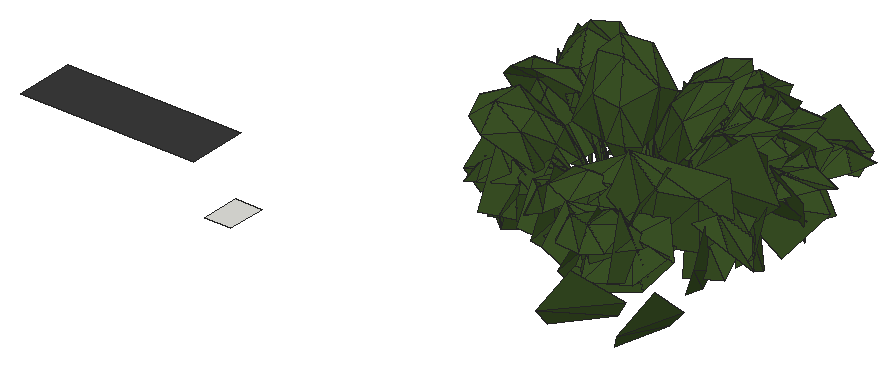
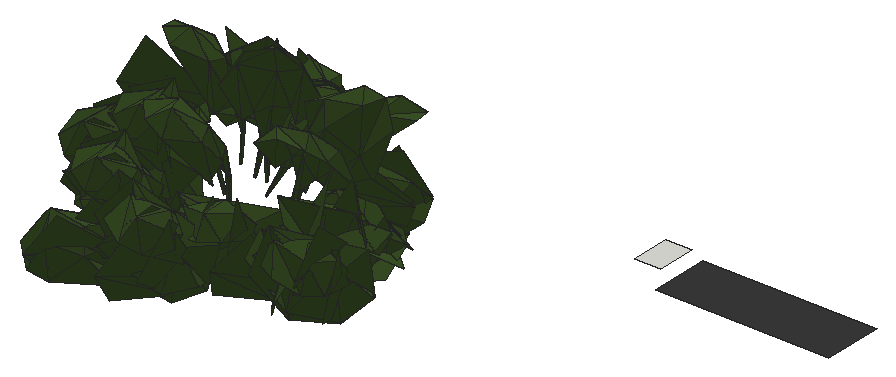
# SketchUp Ruby script. Lengths in inches.
U = 1.inch
M = Sketchup.active_model
def pt(a) = Geom::Point3d.new(a.map { |v| v * U })
def face(e, loops, mat)
  f = e.add_face(loops[0].map { |a| pt(a) })
  loops[1..].each { |l| e.add_face(l.map { |a| pt(a) }).erase! }
  f.material = f.back_material = mat if mat
  f
end
# faces: each face lists its corners as indices into pts; further lists are holes
def faces(e, pts, list, mat = nil) = list.each { |f| face(e, (f[0].is_a?(Array) ? f : [f]).map { |l| l.map { |i| pts[i] } }, mat) }
# xy, xz, yz: faces in a plane at the given z, y or x. An outline is a flat list of corners, or four numbers for a rectangle; further outlines are holes
def ring(l) = l.size == 4 ? [[l[0], l[1]], [l[2], l[1]], [l[2], l[3]], [l[0], l[3]]] : l.each_slice(2).to_a
def flat(e, list, mat, &to3) = list.each { |f| face(e, (f[0].is_a?(Array) ? f : [f]).map { |l| ring(l).map { |u, v| to3.(u, v) } }, mat) }
def xy(e, z, list, mat = nil) = flat(e, list, mat) { |x, y| [x, y, z] }
def xz(e, y, list, mat = nil) = flat(e, list, mat) { |x, z| [x, y, z] }
def yz(e, x, list, mat = nil) = flat(e, list, mat) { |y, z| [x, y, z] }
def lines(e, pts, list) = list.each { |a, b| e.add_line(pt(pts[a]), pt(pts[b])) }
# prism: a flat outline (further loops are holes) pulled along v
def prism(e, loops, v, mat = nil)
  f = face(e, loops, mat); d = Geom::Vector3d.new(v.map { |x| x * U })
  f.pushpull(f.normal.samedirection?(d) ? d.length : -d.length)
end
def box(e, o, s, mat = nil) = prism(e, [[o, [o[0] + s[0], o[1], o[2]], [o[0] + s[0], o[1] + s[1], o[2]], [o[0], o[1] + s[1], o[2]]]], [0, 0, s[2]], mat)
def at(x, y, z, deg = 0) = Geom::Transformation.translation(pt([x, y, z])) * Geom::Transformation.rotation(ORIGIN, Z_AXIS, deg.degrees)
def axes(o, x, y, z) = Geom::Transformation.new([*x, 0, *y, 0, *z, 0, *pt(o).to_a, 1])
def part(name) = M.definitions.add(name)
# library, detail: a bought-in or finely detailed component or shape, given as its bounding box
def library(name, o, s) = part(name).tap { |d| box(d.entities, o, s) }
def detail(e, o, s) = box(e.add_group.entities, o, s)
def put(e, d, t, mat = nil) = e.add_instance(d, t).tap { |i| i.material = mat if mat }
def group(e, t, mat = nil) = e.add_group.tap { |g| g.transformation = t; g.material = mat if mat }.entities
root = M.entities
M.materials.add("AM113_062_Tilia").color = [58, 81, 37]
M.materials.add("[Color M07]").color = [58, 58, 58]
xy(root,620.81,[[1005.08,76.875,1049.99,143.25]])
xy(root,656.55,[[635.92,139.5,935.92,242.3125]],"[Color M07]")
p = [[1488.26,491.22,685.84],[1470.33,571.88,616.22],[1458.61,633.11,690],[1334.86,305.49,619.67],[1391.625,270.38,655.06],[1365.92,294.5625,722.98],
  [1315.2,318.31,702.43],[1301.01,382.23,708.31],[1269.46,349.83,649.08],[1468.55,473.23,668.52],[1471.32,455.52,621.81],[1471.95,459.43,619.89],
  [1472.12,479.33,668.52],[1464.06,473.77,663.09],[1469.125,458.75,620.19],[1549.65,111.21,653.48],[1551.18,136.4,622.06],[1625.28,194.6875,635.39],
  [1581.5,569.83,654.95],[1581.3,541.98,623.84],[1580.58,538.99,627.35],[1555.76,507.45,667.875],[1556.21,492.86,624.24],[1554.3,489.36,625.47],
  [1243.96,537.05,624.62],[1217.14,497.63,657.09],[1243.07,540.83,706.24],[1290.72,590.88,638.93],[1556.28,503.66,674.15],[1558.24,490.84,624.95],
  [1563.01,503.97,676.91],[1583.71,568.81,662.28],[1583.86,540.84,624.87],[1590.32,571.3,662.4375],[1541.83,697.15,663.1875],[1526.4,683.89,626.33],
  [1441.31,645.67,648.45],[1711.43,252.64,709.43],[1697.54,250.96,667.9375],[1662,333.51,628.85],[1661.35,354.26,649.21],[1346.14,511.9,715.51],
  [1327.72,581.9375,629.01],[1282.07,639.52,683.09],[1348.13,547.43,629.25],[1335.29,534.26,653.09],[1389.37,638.25,699.15],[1394,627.73,656.4],
  [1231.01,557.98,751.58],[1251.6,519.09,632.32],[1325.375,499.6,699.71],[1231.08,592.18,653.14],[1574.57,677.58,673.74],[1542.57,657.91,632.77],
  [1572.19,623.15,633.99],[1608.22,714.23,639.1875],[1542.96,290.09,709.29],[1554.42,211.5,633.7],[1559.8,146.17,702.68],[1722.66,477.86,659.14],
  [1678.98,531.82,633.72],[1670.15,531.59,714.6875],[1639.34,563.67,656.82],[1693.67,108.46,664.18],[1674.61,127.09,634.76],[1695.85,219.52,634.04],
  [1712.96,229.3,656.07],[1569.43,621.53,671.65],[1315.94,301.49,634.76],[1369.38,257.5,669.96],[1370.45,307.16,720.57],[1340.08,413.9375,668.15],
  [1280.74,374.8125,651.5],[1329.63,343.92,700.77],[1308.54,471.87,634.8],[1244.51,440.69,650.38],[1269.33,362.61,661.23],[1297.38,416.88,699.34],
  [1337.02,381.32,725.68],[1408.1,373.04,698.34],[1641.15,192.4375,661.92],[1485.7,548.62,676.07],[1493.33,531.125,635.42],[1493.66,527.36,637.49],
  [1459.4,345.02,708.55],[1488.46,269.38,635.86],[1470.08,200.79,695.18],[1436.11,392.38,635.88],[1406.28,385.73,674.23],[1412.9,385.52,677.43],
  [1439.12,393.8,639.24],[1488.29,546.57,682.82],[1496.15,530.625,636.17],[1493.82,550.78,684.54],[1681.41,540.79,764.04],[1659.32,526.72,636.34],
  [1619.97,455.93,693.92],[1729.82,536.63,676.24],[1415.83,381.02,673.47],[1437.8,390.24,637.22],[1445.99,651.32,637.23],[1399.87,632.28,663.58],
  [1445.6875,642.29,718.17],[1515.59,662.1875,657.4375],[1609,448.5,678.25],[1598,431.24,638.73],[1594.87,429.2,640.92],[1274.1875,588,724.35],
  [1329.8,586.84,769.29],[1323.45,636.31,716.625],[1627.78,698.02,686.42],[1642.94,718.39,647.91],[1649.35,717.79,669],[1645.96,691.48,639.38],
  [1568.36,638.77,657.32],[1608.43,445.57,685.24],[1598.95,428.59,639.72],[1614.8,442.95,687.29],[1445.64,655.87,767.97],[1440.8,631.68,639.78],
  [1485.44,561.59,692.13],[1469.01,697.22,679.18],[1228.48,557.13,640.49],[1207.75,512.12,665.06],[1254.89,534.56,708.76],[1282.91,605.98,658.12],
  [1509,556.04,707.76],[1539.51,634.37,641.04],[1537.59,698.13,712.72],[1285.61,359.41,641.44],[1343.48,326.85,677.9],[1331.86,370.95,734.7],
  [1274.27,459,694.77],[1230.86,418.64,662.12],[1281.29,395.8125,715.81],[1441.8125,588.85,642.22],[1380.67,550.67,646.54],[1400.91,546.13,723.81],
  [1446.92,581.53,729.59],[1507.93,561.64,747.36],[1503.37,616.05,703.2],[1626.65,433.54,711.53],[1710.49,442.56,645.39],[1764.2,479.29,715.14],
  [1602.61,375.13,736.48],[1639.9375,316.6875,645.89],[1721.1,307.04,674.03],[1562.79,323.28,646.15],[1560.28,301.26,693.13],[1564.38,307,693.65],
  [1563.74,327.02,648.38],[1568.87,306.3125,688.24],[1565.66,323.6875,646.53],[1353.125,516.4,686.79],[1656.02,648.8125,708.6875],[1674.64,692.49,670.84],
  [1432.22,643.95,679.9],[1571.78,608.95,780.51],[1565.51,604.36,648.81],[1561.13,516.73,686.49],[1620.88,639.375,702.5],[1682.62,311.28,741.96],
  [1405.96,560.97,772.58],[1384.36,530.72,649.5],[1462.1,486.35,679.47],[1391.66,603.83,681.81],[1643.04,587.16,674.75],[1580.5625,618.07,650.66],
  [1568.73,602.65,728.49],[1529.52,624.78,671.32],[1334.67,487.61,687.26],[1354.39,473.34,651.58],[1356.77,470.92,654.56],[1310.49,439.12,725.7],
  [1264.94,401.33,700.87],[1322.63,392.58,652.08],[1399.37,514.43,699.8125],[1337.44,488.54,694.29],[1356.85,474.79,652.34],[1339.12,495.4,694.7],
  [1366.73,579.59,738.91],[1576.61,497.74,701.32],[1649.61,552.72,653.22],[1676.07,599.43,737.56],[1591.26,136.9375,718.13],[1557.67,413.21,697.77],
  [1557.91,398.46,654.22],[1555.51,395.25,655.33],[1388.75,471.01,672.11],[1311.03,530.23,654.22],[1280.125,542.71,754.53],[1585.77,606.67,693],
  [1421.1,264.83,712.85],[1557.43,409.43,704.08],[1559.625,396.2,655.06],[1564.03,408.86,707.27],[1735.41,483.34,682.14],[1698.11,544.21,655.09],
  [1662.0625,520.75,715.01],[1653.45,570.88,668.76],[1311.3125,385.45,776.35],[1359.99,338.83,676.91],[1367.67,429.4375,655.21],[1731.99,377.8,662.9],
  [1669.33,437.34,655.16],[1696.97,413.18,697.4],[1638.3125,406.06,670.76],[1717.95,158.32,719.35],[1610.91,542.06,710.05],[1303.23,438.04,785.74],
  [1247.07,480.625,727.68],[1280.02,436.51,657.11],[1371.11,451.89,662.48],[1240.87,481.17,716.82],[1302.56,364.49,700.02],[1297.08,376.97,657.22],
  [1273.64,320.59,675.82],[1356.08,381.21,659.3],[1552.86,643.14,683.78],[1498.77,656.94,742.58],[1540.86,615.42,779.34],[1567.47,665.41,739.65],
  [1296.78,569.64,729.85],[1369.97,552.86,734.37],[1344.23,620.09,726.67],[1516.38,219,764.9375],[1516.59,166.54,716.65],[1581.02,190.87,658.67],
  [1575.58,194.57,746.38],[1624.62,225.9,743.95],[1645.26,223.14,666.72],[1693.27,438.81,783.98],[1750.28,438.52,745.22],[1708.89,494.03,742.9],
  [1445.74,673.74,659.25],[1401.17,647.92,675.83],[1451.1,629.9,717.74],[1518.24,675.625,680.62],[1371.61,383.33,691.21],[1600.875,525.85,660.27],
  [1660.24,404.05,739.24],[1323.125,322.27,702.34],[1566.68,589.48,725.55],[1513.23,573.85,661.45],[1618.61,483.34,729.83],[1537.95,635.79,686.8],
  [1610.47,595.6,687.74],[1740.63,345.3,678],[1723.95,364.24,716.66],[1459.32,496.78,716.17],[1432.51,500.49,709.2],[1506.42,665.66,729.71],
  [1497.84,379.45,663.36],[1480.69,355.57,703.1875],[1484.6,360.96,706.26],[1498.25,383,666.28],[1407.07,596.07,715.42],[1338.21,294.62,761.84],
  [1333.03,256.62,665.98],[1405.9,283.29,663.82],[1401.74,374.22,684.89],[1526.1,522.45,695.2],[1520.02,594.2,702.7],[1443.72,603.34,664.45],
  [1463.5,557.62,723.91],[1376.25,572.21,669.27],[1410.4375,536.85,720.68],[1413.78,580.09,664.59],[1552.5,570.22,732.43],[1490.31,360.18,703.36],
  [1500.4,379.62,665.15],[1259.71,466.13,670.82],[1264.35,447.85,665.53],[1273.67,396.15,681.16],[1298.38,437.93,733.32],[1284.99,515.18,685.89],
  [1675.28,252.875,709.91],[1634.84,597.41,666.9],[1681.35,631.11,685.1875],[1559.56,526.6,723.57],[1550.86,550.73,710.45],[1444.48,313.51,711.39],
  [1481.8125,505.8,699.76],[1606.64,697.54,735.66],[1281.01,291.8,701.58],[1304.35,299.39,669.27],[1389.67,323.44,712.77],[1350.7,531.85,699.14],
  [1415.13,273.71,739.52],[1427.01,223.68,689.4],[1504.74,245.7,669.56],[1474.13,245.79,748.34],[1521.66,273.39,773.12],[1563.28,272.625,711.46],
  [1405.89,256.02,719.63],[1641.17,414.03,707.03],[1617.71,209.34,791.4],[1629.17,169.65,697.62],[1643.33,243.16,671.1875],[1569.52,292.875,703.625],
  [1504.05,454.65,717.35],[1510.13,447.75,671.32],[1508.98,443.8125,671.41],[1511.89,585.65,714.82],[1505.05,450.13,722.64],[1512.51,446.12,671.83],
  [1596.6875,650.71,701.18],[1511.375,451.35,726.39],[1321.32,468.36,787.75],[1384.3,368.84,716.31],[1394.51,343.2,716.29],[1714.63,381.49,735.92],
  [1619.02,583.45,757.11],[1629.07,522.44,785.5],[1681.4,553.35,757.84],[1639.9,495.77,675.53],[1628.94,492.83,710.47],[1667.28,530.2,732.97],
  [1640.19,541.18,681.94],[1290.7,280.6875,689.27],[1421.75,509.85,676.08],[1406.65,544.09,740.81],[1244.31,541.03,724.9],[1238.58,505.43,681.75],
  [1283.75,510.54,676.08],[1287.15,505.65,713.18],[1380.78,515.875,700.96],[1479.33,573.73,727.26],[1458.6875,587.38,711.51],[1743.32,341.98,699.98],
  [1713.45,339.25,676.53],[1656.1875,414.23,688.98],[1493.18,570.57,737.28],[1492.16,526.59,676.71],[1513.94,578.31,700.89],[1459.89,598.89,676.68],
  [1446.35,638.83,736.35],[1420.98,621.5,686.79],[1287.02,326.22,706.9375],[1581.96,511.74,716.91],[1590.49,634.59,677.1875],[1650.51,594.53,700.5625],
  [1381.18,331.9,727.2],[1681.24,336.31,755.66],[1721.25,315.6875,713.07],[1627.13,468.95,728.18],[1560.92,563.1,678.63],[1565.92,597.61,745.6875],
  [1539.53,602.02,692.4375],[1408.9,412.64,723.88],[1420.31,416.14,678.92],[1423.27,413.31,679.14],[1413.07,411.29,729.51],[1422.82,417.49,679.72],
  [1582.44,512.34,811.29],[1580.82,507.9,679.35],[1563.47,421.8125,716.71],[1386.07,473.98,679.42],[1638.13,535.62,736.64],[1502.38,262.01,715.72],
  [1501.96,189.78,717.66],[1577.57,175.61,679.7],[1561.26,220.09,742.39],[1615.99,236.12,741.43],[1647.48,200.28,687.77],[1414.68,417.36,733.7],
  [1505.18,628.25,741],[1573.66,638.79,743.23],[1425.15,419.96,680.92],[1403.63,428.09,727.22],[1410.3125,430.4,727.33],[1427.97,423.09,681.41],
  [1323.58,387.09,707.13],[1589.52,396.21,705.28],[1558.26,390.04,681.42],[1555.69,391.04,685.35],[1413.93,425.46,726.22],[1427.54,419.15,682.8125],
  [1229.79,590.89,696.18],[1722.08,537.78,718.14],[1730.17,420.16,749.96],[1687.16,474.19,742.56],[1654.29,480.79,710.4],[1597.46,519.52,682.2],
  [1580.64,506.21,759.15],[1546.99,532.99,699.45],[1260.66,576.39,758.79],[1589.66,395.03,713.1],[1557.53,387.59,683.24],[1592.79,388.74,714.13],
  [1509.64,364.38,732.16],[1500.48,377.7,684.39],[1499.53,381.35,686.86],[1503.78,365.3,729.91],[1497.3,379.48,686.84],[1506.1,572.52,720.04],
  [1360.58,301.51,737.93],[1405.93,290.09,718.22],[1400.22,327.47,685.16],[1418.68,319.82,691.9],[1414.29,247.875,685.76],[1494.65,229.8125,685.68],
  [1463.28,272.45,740.47],[1514.91,284.33,767.73],[1558.07,248.74,729.52],[1439.8,570.31,767.29],[1311.7,490.55,760.52],[1372.76,513.92,767.99],
  [1326.48,558.19,758.76],[1384.54,488.45,731.66],[1466.18,690.43,721.22],[1511.42,369.8125,737.53],[1639.41,444.8,723.14],[1310.53,509.9375,731.28],
  [1676.18,236.72,721.06],[1570.93,280.55,739.48],[1597.38,274.79,732.55],[1577,493.41,756.08],[1524.55,484.59,688.52],[1614.26,381.38,763.82],
  [1556.17,542.89,715.47],[1662.25,433.51,710.24],[1322.59,269.31,703.5],[1304.5,307.58,721.44],[1575.71,401.03,732.55],[1657.11,445.67,689.34],
  [1686.125,488.96,775.3125],[1454.87,311.85,690.51],[1422.08,262.6,690.57],[1430.72,263.45,735.46],[1459.47,328.41,721.11],[1449.54,211.88,722.42],
  [1350.64,340.95,733.98],[1252.76,625.59,725.21],[1269.57,609.48,691.37],[1271.06,515.01,702.03],[1556.47,345.64,755.82],[1611.375,631.08,742.41],
  [1427.52,361.25,735.16],[1433.15,376.6,692.57],[1435.51,379.7,694.25],[1547.91,274.36,722.11],[1431.44,378.93,693.13],[1420.25,365.74,743.39],
  [1427.13,364.93,741.55],[1332.92,524.47,723.47],[1390.04,383.54,746.875],[1470.29,252.18,788.62],[1258.55,595.92,739.59],[1246.65,621.57,704.6],
  [1245.47,376.42,734.64],[1263.55,371.41,696.41],[1355.92,391.37,706.86],[1619.2,267.12,710.98],[1671.02,316.08,696.55],[1669.24,314.79,778.27],
  [1700.35,353.94,728.48],[1606.375,361.5,773.91],[1678.99,392.03,697.21],[1747.73,392.13,760.83],[1536.02,255.7,697.36],[1509.44,205.12,717.18],
  [1530.39,209.26,754.35],[1676.24,393.54,734.96],[1561.75,432,753.64],[1556.83,457,739.95],[1252.58,452.9,697.91],[1282.14,520.01,714.125],
  [1366.7,327.88,740.77],[1542.12,378.08,698.3],[1542.07,372.75,749.96],[1542.78,378.36,746.72],[1546.28,378.74,698.85],[1544.7,381.16,699.4],
  [1569.02,353.05,780.82],[1583.47,279,698.73],[1622.16,219.33,757.83],[1607.64,266.04,698.9],[1618.89,227.66,761.01],[1647.62,255.23,723.76],
  [1548.46,370.65,752.78],[1522.68,496.76,741.73],[1337.5,487.6,742.67],[1446.125,534.43,745.24],[1352.16,555.26,746.73],[1727.53,391.96,759.89],
  [1609.21,556.34,749.54],[1672.07,527.56,755.8],[1471.28,620.81,723.6],[1400.65,598.5,722.74],[1597.47,585.32,787.7],[1393.6,325.8125,745.89],
  [1310.17,321.26,774.4],[1261.34,503.4,729.42],[1316.83,590.9,752.28],[1343.07,546.61,702.47],[1343.25,603.09,725.22],[1583.23,203.34,784.97],
  [1475.94,332.04,748.92],[1533.52,629.02,765.22],[1528.2,586.62,703.17],[1562.48,626.51,738.11],[1502.15,324.63,754.68],[1631.36,539.12,774.32],
  [1609.43,513.09,703.88],[1656.57,523.98,747.82],[1287.82,632.37,721.92],[1630.89,400.02,734.69],[1646.34,298.35,705.47],[1365.41,401.49,735.34],
  [1582.23,414.29,748.47],[1662.76,431.8,707.69],[1714.03,423.53,744.28],[1701.59,451.2,768.96],[1480.16,650.94,775.42],[1418.93,308.17,755.53],
  [1569.67,467.76,708.84],[1576.52,501.67,776.13],[1553.07,509.23,721.21],[1661.64,487.26,736.67],[1608.41,534.73,709.34],[1645.96,281.41,756.51],
  [1626.78,480.72,791.06],[1627.57,419.07,820.1],[1684.53,442.6875,795.93],[1576.7,559.5,758.26],[1660.92,493.08,753.18],[1576.97,278.69,838.93],
  [1580.31,227.25,789.03],[1633.49,271.1875,796.99],[1579.76,297.99,769.03],[1694.13,508.8,774.34],[1476.33,614.63,753.59],[1663.45,306.89,742.45],
  [1281.34,543.14,746.78],[1621.82,374.29,737.53],[1547.88,157.98,737.03],[1500.42,464.85,776.86],[1487.33,488.28,768.56],[1716.34,508.28,760.59],
  [1748.27,516.72,733.37],[1475.08,290.36,773.43],[1626.05,528.86,775.86],[1490.9375,670.2,761.27],[1498.125,702.52,734.24],[1580.38,240.6,765.7],
  [1623.43,347.55,722.23],[1489.65,202.54,744.62],[1438.75,591.53,751.17],[1426.71,622.73,724.83],[1620.22,173.86,738.78],[1394.93,412.45,782.29],
  [1368.63,411.87,771.54],[1251.85,575.9,788.86],[1392.99,431.07,780.58],[1410.22,412.41,794.52],[1525.875,456.25,770.07],[1373.72,428.93,755.65],
  [1521.1,316.6875,727.61],[1511.43,274.8,786.3],[1550.24,301.78,768.71],[1676.52,374.3,786.11],[1576.55,281.34,778.03],[1512.15,351.21,787.26],
  [1485.52,344.47,790.69],[1604.48,485.57,820.18],[1750.48,474.32,751.11],[1414.58,431.24,778.16],[1536.82,683.2,748.45],[1288.53,417.93,781.64],
  [1415.96,341.88,788.92],[1421.51,316.89,775.6],[1473.92,232.6875,769.74],[1613.79,455.09,782.86],[1671.98,418.33,793.28],[1592.09,152.01,738.65],
  [1632.47,435.25,809.08],[1610.11,411.94,737.28],[1656.48,416.79,784.28],[1524.45,375.31,781.86],[1355.87,410.12,738.07],[1301.29,397.03,762.22],
  [1315.3,407.9,802.4375],[1582.58,182.9,767.24],[1540.34,326.47,800.96],[1581.67,462.55,789.41],[1395.95,272.59,805.96],[1425.47,264.82,756.21],
  [1412.21,307.11,741.96],[1496.125,507.25,741.95],[1489.64,530.58,816.41],[1465.93,537.94,761.63],[1617.98,596.83,778.18],[1643.53,622.41,758.68],
  [1397.0625,360.5,780.24],[1516.64,222.16,760.66],[1357.3,429.15,744.625],[1329.58,432.05,816.92],[1315.2,415.96,759.9],[1544.7,374.36,807.58],
  [1541.49,401.68,810.46],[1664.46,583.9,769.54],[1564.69,359.27,793.33],[1371.67,412.3125,826.96],[1346.04,247.52,794.87],[1647.02,282.62,831.52],
  [1308.8125,483.76,828.99],[1694.13,396.48,852.01],[1526.59,572.38,827.92],[1564.67,483.32,839.93],[1553,465.2,761.71],[1594.01,478.2,814.125],
  [1298.16,357.82,825.26],[1371,364.18,763.65],[1319.34,360.64,800.57],[1339.3,340.84,829.31],[1507.88,494.28,821.12],[1369.84,431.37,825.29],
  [1404.51,476.16,849.43],[1419.51,459.66,771.57],[1423.89,500.53,826.47],[1390.76,311.7,819.26],[1626.67,494.23,812.03],[1656.1,516.125,794.25],
  [1393.22,384.6,853.75],[1436.96,373.22,828.7],[1416.51,386.43,778.84],[1463.74,343.84,857.66],[1434.05,334,808.68],[1463.05,361.55,780.21],
  [1501.9375,354.04,844.76],[1532.59,402.14,867.27],[1521.3,404.28,785.6],[1592.98,359.41,783.49],[1636.96,343.54,830.26],[1612.47,352.39,862.08],
  [1671.33,475.26,806.49],[1537.03,434.46,848.04],[1556.34,421.6,790.27],[1561.02,426.59,870.53],[1540.79,454.75,825.52],[1563.92,386.96,858.71],
  [1314.64,261.25,807.37],[1342.375,281.64,831.54],[1299.71,302.54,817.67],[1327.6875,335.22,857.1],[1336.59,373.37,858.25],[1440.51,383.56,899.97],
  [1587.2,533.68,850.86],[1538.65,535.22,855.57],[1345.75,476.55,859.77],[1611.49,447.35,889.41],[1369.59,519.03,859.23],[1558.89,568.02,846.4375],
  [1362.83,337.62,863.89],[1326.45,509.875,850.41],[1652.92,386.01,886.16],[1484.87,382.97,905.37],[1497.8,429.73,910.9],[1608.86,403.67,900.24],
  [1640,427.46,899.43],[1458.71,409.6,920.73]]
faces(root,p,[[0,1,2],[3,4,5],[5,6,3],[7,8,3],[3,6,7],[9,10,11],[11,12,9],[13,14,10],
  [10,9,13],[15,16,17],[18,19,20],[21,22,23],[24,25,26],[27,24,26],[28,23,29],[29,30,28],
  [31,20,32],[32,33,31],[23,28,21],[34,35,36],[20,31,18],[37,38,39],[39,40,37],[41,42,43],
  [44,45,46],[46,47,44],[48,49,50],[48,51,49],[52,53,54],[55,53,52],[56,57,58],[59,60,61],
  [60,62,61],[63,64,65],[65,66,63],[54,67,52],[68,69,70],[71,72,68],[68,73,71],[70,73,68],
  [74,75,76],[76,77,74],[78,79,74],[74,77,78],[17,80,15],[81,82,83],[84,85,86],[87,88,89],
  [89,90,87],[91,83,92],[92,93,91],[94,95,96],[94,97,95],[98,99,90],[100,101,102],[103,100,102],
  [83,91,81],[104,105,106],[26,107,27],[27,107,108],[108,109,27],[90,89,98],[110,55,52],[111,55,110],
  [112,113,114],[115,106,116],[116,117,115],[118,119,120],[118,121,119],[122,123,124],[125,122,124],[106,115,104],
  [126,127,128],[129,130,131],[132,133,129],[129,134,132],[131,134,129],[135,136,137],[137,138,135],[139,140,135],
  [135,138,139],[141,142,143],[144,145,146],[147,148,149],[149,150,147],[151,152,150],[136,153,137],[111,110,154],
  [154,155,111],[150,149,151],[36,156,34],[157,158,159],[157,160,158],[40,161,37],[162,163,164],[162,165,163],
  [166,167,168],[167,169,168],[170,171,172],[173,174,175],[173,175,176],[177,172,178],[178,179,177],[45,180,46],
  [181,182,183],[80,184,15],[185,186,187],[188,189,190],[172,177,170],[18,31,191],[191,67,18],[4,192,5],
  [193,187,194],[194,195,193],[196,197,198],[197,199,198],[200,201,202],[203,204,205],[205,204,206],[187,193,185],
  [66,207,63],[61,62,208],[209,210,211],[209,211,212],[26,25,213],[214,215,216],[217,215,214],[114,218,112],
  [103,219,220],[220,221,103],[102,219,103],[124,222,125],[223,224,125],[125,222,223],[225,226,227],[227,228,225],
  [229,228,227],[227,230,229],[231,232,59],[59,233,231],[61,233,59],[234,235,236],[237,234,236],[214,238,217],
  [198,239,240],[198,199,239],[76,241,78],[78,77,76],[242,243,244],[242,245,243],[191,31,33],[33,246,191],
  [247,203,248],[248,203,205],[13,9,249],[249,250,13],[156,251,34],[252,253,254],[254,255,252],[102,101,256],
  [257,258,259],[257,259,260],[261,262,263],[263,264,261],[263,265,266],[266,264,263],[236,267,268],[236,235,267],
  [269,270,255],[124,123,271],[272,273,274],[275,272,274],[255,254,269],[230,276,229],[154,246,277],[277,278,154],
  [21,28,279],[279,280,21],[71,73,70],[70,281,71],[249,9,12],[12,282,249],[218,283,112],[284,285,286],
  [265,287,266],[288,289,290],[290,291,288],[292,291,290],[290,293,292],[69,294,70],[206,295,205],[124,271,223],
  [154,278,155],[296,297,298],[296,298,299],[300,301,302],[168,169,303],[302,304,300],[304,302,305],[306,67,191],
  [306,52,67],[305,307,304],[308,188,190],[309,310,98],[98,89,309],[306,110,52],[311,144,146],[88,238,309],
  [309,89,88],[279,28,30],[166,312,313],[313,314,166],[168,312,166],[315,316,317],[317,318,315],[214,216,319],
  [320,250,321],[322,323,324],[324,325,322],[321,326,320],[81,91,327],[327,328,81],[329,330,331],[332,282,333],
  [333,334,332],[335,328,336],[336,337,335],[200,338,201],[30,339,279],[340,245,242],[341,340,242],[130,342,131],
  [343,344,247],[247,248,343],[104,115,345],[345,316,104],[346,280,347],[347,348,346],[349,350,351],[351,352,349],
  [352,351,353],[354,355,356],[266,287,357],[266,357,261],[354,358,355],[359,360,361],[361,362,359],[363,362,361],
  [361,364,363],[353,365,352],[237,366,268],[268,367,237],[236,366,237],[368,369,370],[370,371,368],[274,273,372],
  [373,374,375],[376,377,371],[371,370,376],[378,323,322],[379,318,317],[240,380,196],[196,381,240],[198,381,196],
  [382,383,384],[383,385,384],[327,91,93],[386,41,43],[387,375,388],[388,389,387],[390,391,392],[391,390,393],
  [393,394,391],[93,395,327],[396,397,398],[398,310,396],[345,115,117],[375,387,373],[399,400,401],[401,402,399],
  [403,402,401],[401,404,403],[405,0,2],[274,406,275],[275,406,407],[407,408,275],[154,110,306],[137,153,409],
  [410,337,336],[392,411,390],[117,412,345],[413,325,170],[170,177,413],[306,191,246],[246,154,306],[364,414,363],
  [415,416,151],[151,149,415],[417,418,419],[417,420,418],[331,421,329],[319,422,423],[319,423,214],[424,425,426],
  [427,428,429],[429,430,427],[429,428,431],[238,214,432],[432,309,238],[433,434,435],[399,402,403],[403,436,399],
  [437,348,347],[438,439,440],[148,441,415],[415,149,148],[442,443,444],[444,440,442],[440,444,438],[413,177,179],
  [179,445,413],[131,446,132],[132,134,131],[447,84,86],[261,264,266],[448,378,322],[449,378,448],[450,451,452],
  [453,454,455],[454,456,455],[457,458,459],[460,461,462],[462,441,460],[463,248,205],[463,205,295],[185,193,464],
  [464,465,185],[466,174,173],[467,466,173],[78,468,79],[469,470,471],[470,469,472],[471,473,469],[474,475,476],
  [477,416,478],[478,479,477],[472,480,470],[384,385,481],[176,482,173],[467,482,176],[483,249,282],[282,332,483],
  [176,484,467],[214,423,432],[421,485,329],[341,486,244],[244,487,341],[242,486,341],[332,334,488],[489,326,321],
  [490,181,183],[286,491,284],[491,492,284],[435,493,433],[241,468,78],[7,6,5],[494,445,495],[495,496,494],
  [497,56,58],[253,430,498],[498,254,253],[499,395,500],[500,501,499],[498,502,269],[269,254,498],[423,422,396],
  [422,397,396],[503,339,504],[504,505,503],[464,193,195],[494,506,449],[449,448,494],[373,387,507],[507,295,373],
  [363,508,359],[363,414,508],[26,213,108],[108,107,26],[452,509,450],[463,295,507],[274,372,407],[195,510,464],
  [511,512,513],[513,412,511],[514,126,128],[5,515,7],[516,465,517],[517,518,516],[223,222,124],[483,250,249],
  [483,321,250],[519,520,417],[520,420,417],[229,276,521],[61,208,231],[382,522,523],[523,524,382],[384,522,382],
  [525,280,279],[525,347,280],[526,316,345],[526,317,316],[527,528,453],[453,529,527],[455,529,453],[70,294,281],
  [293,530,292],[531,141,143],[532,328,327],[532,336,328],[5,192,515],[343,533,344],[507,387,389],[534,322,325],
  [534,325,413],[389,535,507],[173,482,467],[231,233,61],[168,303,313],[240,381,198],[102,256,220],[359,362,363],
  [432,396,310],[432,310,309],[343,248,463],[525,279,339],[339,503,525],[462,461,536],[300,304,537],[537,538,300],
  [268,366,236],[539,379,317],[540,379,539],[220,219,102],[395,499,532],[532,327,395],[430,429,541],[541,498,430],
  [542,518,517],[543,410,336],[544,410,543],[432,423,396],[494,496,506],[441,462,545],[545,415,441],[546,533,343],
  [343,535,546],[429,431,547],[537,304,307],[548,489,321],[549,489,548],[526,345,412],[412,513,526],[534,413,445],
  [445,494,534],[332,488,549],[550,479,478],[137,409,139],[139,138,137],[349,352,551],[551,552,349],[549,548,332],
  [534,448,322],[493,553,433],[244,486,242],[554,555,376],[376,370,554],[307,556,537],[131,342,446],[369,557,554],
  [554,370,369],[558,502,559],[559,560,558],[455,456,561],[313,312,168],[404,562,403],[551,352,365],[563,564,393],
  [393,390,563],[563,390,411],[545,478,416],[545,416,415],[565,424,426],[526,539,317],[407,406,274],[513,566,540],
  [540,539,513],[365,567,551],[544,543,499],[499,568,544],[509,569,450],[463,507,535],[535,343,463],[570,571,438],
  [438,444,570],[547,572,429],[429,572,541],[532,543,336],[519,573,419],[419,574,519],[417,573,519],[462,536,575],
  [576,510,577],[577,578,576],[332,548,483],[411,579,563],[580,581,582],[582,557,580],[499,501,568],[575,583,462],
  [575,550,583],[583,550,478],[288,291,292],[292,584,288],[494,448,534],[585,465,464],[585,517,465],[483,548,321],
  [570,444,443],[384,481,523],[586,587,588],[588,571,586],[589,538,590],[590,591,589],[592,437,347],[593,437,592],
  [443,594,570],[225,228,229],[229,521,225],[513,512,566],[547,595,572],[596,552,597],[597,598,596],[525,592,347],
  [471,470,599],[599,600,471],[503,505,601],[585,464,510],[510,576,585],[541,502,498],[599,470,480],[480,602,599],
  [513,539,526],[499,543,532],[462,583,545],[541,559,502],[557,582,603],[603,554,557],[403,562,436],[419,573,417],
  [604,587,586],[605,474,476],[503,592,525],[593,592,503],[503,601,593],[523,522,384],[606,598,597],[572,595,559],
  [595,560,559],[607,457,459],[545,583,478],[608,591,590],[609,556,610],[610,611,609],[582,581,612],[613,614,615],
  [615,594,613],[616,538,537],[616,590,538],[292,530,584],[541,572,559],[616,537,556],[556,609,616],[617,597,552],
  [617,552,551],[618,567,619],[619,620,618],[621,586,571],[621,571,570],[622,542,517],[623,542,622],[585,622,517],
  [617,551,567],[567,618,617],[527,529,455],[455,561,527],[624,625,626],[626,555,624],[594,615,621],[621,570,594],
  [627,628,629],[629,564,627],[603,555,554],[630,563,579],[579,631,630],[631,579,632],[633,634,635],[635,602,633],
  [576,578,636],[632,637,631],[630,564,563],[576,622,585],[638,600,639],[639,640,638],[630,627,564],[602,635,641],
  [641,599,602],[623,622,576],[576,636,623],[603,624,555],[642,604,643],[643,604,586],[615,614,644],[582,612,645],
  [645,646,582],[582,646,603],[621,643,586],[615,644,642],[642,643,615],[641,600,599],[647,628,627],[641,639,600],
  [609,611,648],[616,649,590],[649,608,590],[617,650,597],[650,606,597],[615,643,621],[609,649,616],[618,650,617],
  [651,640,639],[618,620,652],[603,646,624],[653,608,649],[654,625,624],[655,606,650],[635,634,656],[653,649,609],
  [609,648,653],[630,657,627],[631,657,630],[631,637,658],[618,652,655],[655,650,618],[646,654,624],[645,654,646],
  [657,647,627],[635,659,641],[641,659,639],[660,659,635],[635,656,660],[661,657,631],[631,658,661],[659,651,639],
  [660,651,659],[661,647,657]],"AM113_062_Tilia")
